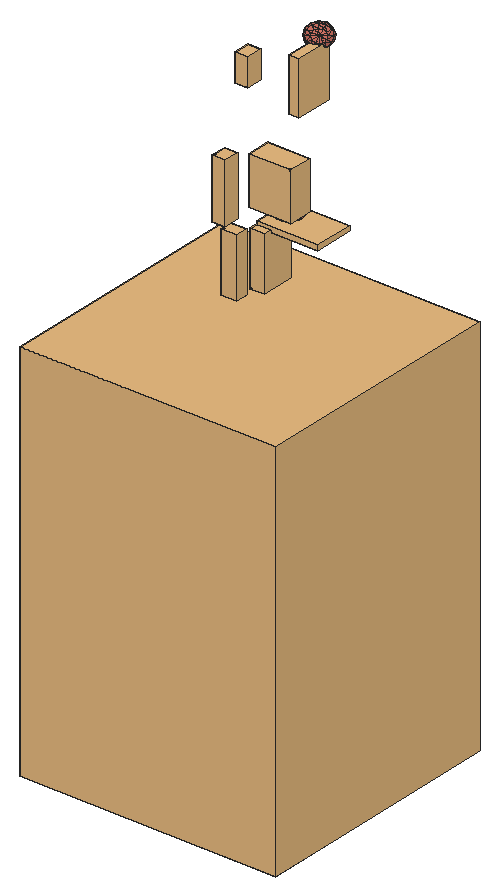
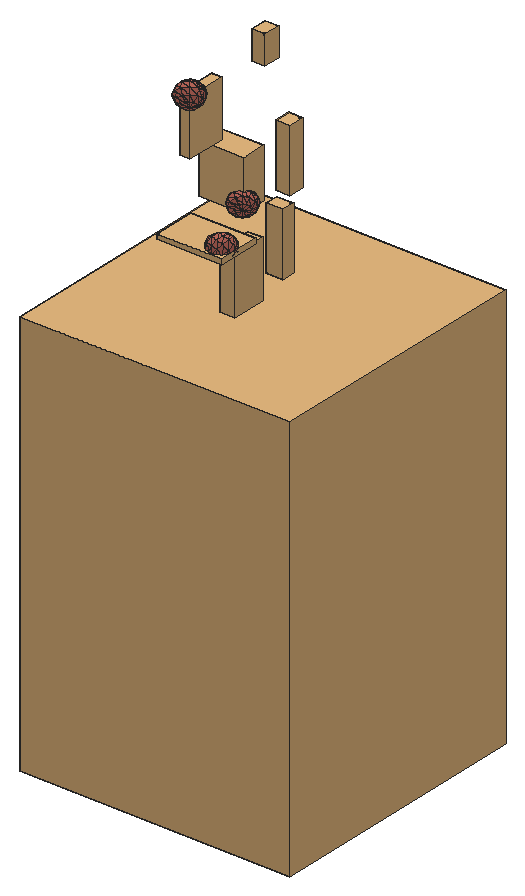
# SketchUp Ruby script. Lengths in inches.
U = 1.inch
M = Sketchup.active_model
def pt(a) = Geom::Point3d.new(a.map { |v| v * U })
def face(e, loops, mat)
  f = e.add_face(loops[0].map { |a| pt(a) })
  loops[1..].each { |l| e.add_face(l.map { |a| pt(a) }).erase! }
  f.material = f.back_material = mat if mat
  f
end
# faces: each face lists its corners as indices into pts; further lists are holes
def faces(e, pts, list, mat = nil) = list.each { |f| face(e, (f[0].is_a?(Array) ? f : [f]).map { |l| l.map { |i| pts[i] } }, mat) }
# xy, xz, yz: faces in a plane at the given z, y or x. An outline is a flat list of corners, or four numbers for a rectangle; further outlines are holes
def ring(l) = l.size == 4 ? [[l[0], l[1]], [l[2], l[1]], [l[2], l[3]], [l[0], l[3]]] : l.each_slice(2).to_a
def flat(e, list, mat, &to3) = list.each { |f| face(e, (f[0].is_a?(Array) ? f : [f]).map { |l| ring(l).map { |u, v| to3.(u, v) } }, mat) }
def xy(e, z, list, mat = nil) = flat(e, list, mat) { |x, y| [x, y, z] }
def xz(e, y, list, mat = nil) = flat(e, list, mat) { |x, z| [x, y, z] }
def yz(e, x, list, mat = nil) = flat(e, list, mat) { |y, z| [x, y, z] }
def lines(e, pts, list) = list.each { |a, b| e.add_line(pt(pts[a]), pt(pts[b])) }
# prism: a flat outline (further loops are holes) pulled along v
def prism(e, loops, v, mat = nil)
  f = face(e, loops, mat); d = Geom::Vector3d.new(v.map { |x| x * U })
  f.pushpull(f.normal.samedirection?(d) ? d.length : -d.length)
end
def box(e, o, s, mat = nil) = prism(e, [[o, [o[0] + s[0], o[1], o[2]], [o[0] + s[0], o[1] + s[1], o[2]], [o[0], o[1] + s[1], o[2]]]], [0, 0, s[2]], mat)
def at(x, y, z, deg = 0) = Geom::Transformation.translation(pt([x, y, z])) * Geom::Transformation.rotation(ORIGIN, Z_AXIS, deg.degrees)
def axes(o, x, y, z) = Geom::Transformation.new([*x, 0, *y, 0, *z, 0, *pt(o).to_a, 1])
def part(name) = M.definitions.add(name)
# library, detail: a bought-in or finely detailed component or shape, given as its bounding box
def library(name, o, s) = part(name).tap { |d| box(d.entities, o, s) }
def detail(e, o, s) = box(e.add_group.entities, o, s)
def put(e, d, t, mat = nil) = e.add_instance(d, t).tap { |i| i.material = mat if mat }
def group(e, t, mat = nil) = e.add_group.tap { |g| g.transformation = t; g.material = mat if mat }.entities
root = M.entities
M.materials.add("green").color = [174, 139, 102]
M.materials.add("st tile").color = [196, 179, 155]
M.materials.add("vio").color = [206, 114, 100]
c1 = library("3DGeom~165_Defintion",[-129.92,-500,-108.02],[259.84,1000,216.04])
c2 = part("3DGeom~166_Defintion")
p = [[102.48,500,-82.55],[119.68,491.3,-106.9],[111.55,493.01,-108.02],[102.48,500,-82.55],[111.55,493.01,-108.02],[104.2,495.34,-104.9],
  [102.48,500,-82.55],[126.4,490.68,-101.84],[119.68,491.3,-106.9],[102.48,500,-82.55],[104.2,495.34,-104.9],[99.59,497.67,-98.37],
  [102.48,500,-82.55],[129.92,491.3,-94.2],[126.4,490.68,-101.84],[102.48,500,-82.55],[99.59,497.67,-98.37],[98.96,499.375,-90.19],
  [102.48,500,-82.55],[129.29,493.01,-86.02],[129.92,491.3,-94.2],[102.48,500,-82.55],[124.6875,495.34,-79.5],[129.29,493.01,-86.02],
  [102.48,500,-82.55],[117.33,497.67,-76.375],[124.6875,495.34,-79.5],[102.48,500,-82.55],[109.21,499.375,-77.49],[117.33,497.67,-76.375],
  [-108.37,-495.57,69.37],[-118.11,-500,95.38],[-120.78,-498.52,79.375],[-93.3,-494.09,75.36],[-118.11,-500,95.38],[-108.37,-495.57,69.37],
  [-108.37,-495.57,69.37],[-120.78,-498.52,79.375],[-115.95,-497.04,72.67],[-93.3,-494.09,75.36],[-108.37,-495.57,69.37],[-100.08,-494.49,70.35],
  [-90.63,-495.57,91.37],[-118.11,-500,95.38],[-93.3,-494.09,75.36],[-90.63,-495.57,91.37],[-93.3,-494.09,75.36],[-89.84,-494.49,83.05],
  [-118.11,-500,95.38],[-121.57,-499.6,87.6875],[-120.78,-498.52,79.375],[-103.04,-498.52,101.375],[-118.11,-500,95.38],[-90.63,-495.57,91.37],
  [-103.04,-498.52,101.375],[-90.63,-495.57,91.37],[-95.46,-497.04,98.07],[-118.11,-500,95.38],[-103.04,-498.52,101.375],[-111.33,-499.6,100.39]]
faces(c2.entities,p,[[0,1,2],[3,4,5],[6,7,8],[9,10,11],[12,13,14],[15,16,17],[18,19,20],[21,22,23],
  [24,25,26],[27,28,29],[30,31,32],[33,34,35],[36,37,38],[39,40,41],[42,43,44],[45,46,47],
  [48,49,50],[51,52,53],[54,55,56],[57,58,59]],"green")
c3 = library("3DGeom~177_Defintion",[-102.18,-500,-134.58],[204.36,1000,269.16])
c4 = part("3DGeom~178_Defintion")
p = [[77.2,500,-106.58],[95.25,490.68,-131.46],[87.43,491.3,-134.58],[77.2,500,-106.58],[87.43,491.3,-134.58],[79.3,493.01,-133.53],
  [77.2,500,-106.58],[79.3,493.01,-133.53],[73.02,495.34,-128.6],[77.2,500,-106.58],[100.64,491.3,-125],[95.25,490.68,-131.46],
  [77.2,500,-106.58],[73.02,495.34,-128.6],[70.28,497.67,-121.1],[77.2,500,-106.58],[102.18,493.01,-116.9375],[100.64,491.3,-125],
  [77.2,500,-106.58],[70.28,497.67,-121.1],[71.81,499.375,-113.04],[77.2,500,-106.58],[99.43,495.34,-109.4375],[102.18,493.01,-116.9375],
  [77.2,500,-106.58],[93.15,497.67,-104.5],[99.43,495.34,-109.4375],[77.2,500,-106.58],[85.02,499.375,-103.46],[93.15,497.67,-104.5],
  [-70.48,-494.09,97.03],[-86.6,-495.57,95.18],[-78.34,-494.49,93.96],[-86.6,-495.57,95.18],[-89.2,-500,122.83],[-95.96,-498.52,108.09],
  [-70.48,-494.09,97.03],[-89.2,-500,122.83],[-86.6,-495.57,95.18],[-86.6,-495.57,95.18],[-95.96,-498.52,108.09],[-93.05,-497.04,100.35],
  [-63.72,-495.57,111.78],[-89.2,-500,122.83],[-70.48,-494.09,97.03],[-63.72,-495.57,111.78],[-70.48,-494.09,97.03],[-65.13,-494.49,103.55],
  [-89.2,-500,122.83],[-94.55,-499.6,116.32],[-95.96,-498.52,108.09],[-73.08,-498.52,124.68],[-89.2,-500,122.83],[-63.72,-495.57,111.78],
  [-73.08,-498.52,124.68],[-63.72,-495.57,111.78],[-66.63,-497.04,119.51],[-89.2,-500,122.83],[-73.08,-498.52,124.68],[-81.34,-499.6,125.9]]
faces(c4.entities,p,[[0,1,2],[3,4,5],[6,7,8],[9,10,11],[12,13,14],[15,16,17],[18,19,20],[21,22,23],
  [24,25,26],[27,28,29],[30,31,32],[33,34,35],[36,37,38],[39,40,41],[42,43,44],[45,46,47],
  [48,49,50],[51,52,53],[54,55,56],[57,58,59]],"green")
c5 = library("3DGeom~138_Defintion",[-301.73,-500,-131.06],[603.46,1000,262.12])
c6 = part("3DGeom~139_Defintion")
p = [[272.8,-500,-99.27],[285.64,-496.58,-110.875],[273.61,-494.75,-82.625],[285.64,-496.58,-110.875],[272.8,-500,-99.27],[278.1,-499.36,-106.75],
  [273.61,-494.75,-82.625],[285.64,-496.58,-110.875],[287.25,-486.08,-77.6],[285.64,-496.58,-110.875],[293.39,-492.38,-110.55],[299.28,-487.9,-105.84],
  [300.09,-482.66,-89.21],[285.64,-496.58,-110.875],[299.28,-487.9,-105.84],[287.25,-486.08,-77.6],[285.64,-496.58,-110.875],[300.09,-482.66,-89.21],
  [300.09,-482.66,-89.21],[299.28,-487.9,-105.84],[301.73,-484.35,-98.03],[272.8,-500,-99.27],[273.61,-494.75,-82.625],[271.16,-498.3125,-90.4375],
  [287.25,-486.08,-77.6],[300.09,-482.66,-89.21],[294.79,-483.3,-81.72],[273.61,-494.75,-82.625],[287.25,-486.08,-77.6],[279.5,-490.28,-77.93],
  [-291.23,494.98,97.6],[-301.04,485.9375,118.13],[-296.26,485.84,125.99],[-291.23,494.98,97.6],[-296.26,485.84,125.99],[-288.67,487.64,130.72],
  [-291.23,494.98,97.6],[-301.73,487.91,109.26],[-301.04,485.9375,118.13],[-291.23,494.98,97.6],[-288.67,487.64,130.72],[-280.29,490.86,131.0625],
  [-291.23,494.98,97.6],[-298.14,491.22,101.74],[-301.73,487.91,109.26],[-291.23,494.98,97.6],[-280.29,490.86,131.0625],[-273.38,494.625,126.92],
  [-291.23,494.98,97.6],[-273.38,494.625,126.92],[-269.79,497.9375,119.41],[-291.23,494.98,97.6],[-270.48,499.9,110.54],[-275.26,500,102.68],
  [-291.23,494.98,97.6],[-275.26,500,102.68],[-282.85,498.2,97.95],[-291.23,494.98,97.6],[-269.79,497.9375,119.41],[-270.48,499.9,110.54]]
faces(c6.entities,p,[[0,1,2],[3,4,5],[6,7,8],[9,10,11],[12,13,14],[15,16,17],[18,19,20],[21,22,23],
  [24,25,26],[27,28,29],[30,31,32],[33,34,35],[36,37,38],[39,40,41],[42,43,44],[45,46,47],
  [48,49,50],[51,52,53],[54,55,56],[57,58,59]],"green")
c7 = part("3DGeom~203_Defintion")
p = [[282.28,-215.46,-337.03],[49.88,-186.59,-454.85],[87.7,0,-500],[282.28,-215.46,-337.03],[325.95,0,-389.16],[-174.05,0,-476.86],
  [-195.89,107.73,-450.79],[49.88,186.59,-454.85],[325.95,0,-389.16],[-195.89,-107.73,-450.79],[-389.16,0,-325.95],[-389.16,0,-325.95],
  [162.97,-373.1875,-194.58],[-53.44,-323.1875,-331.49],[162.97,-373.1875,-194.58],[282.28,-215.46,-337.03],[325.95,0,-389.16],[282.28,215.46,-337.03],
  [-255.54,186.59,-379.57],[-255.54,186.59,-379.57],[-53.44,323.19,-331.49],[282.28,215.46,-337.03],[-53.44,323.19,-331.49],[-255.54,-186.59,-379.57],
  [-389.16,0,-325.95],[-255.54,186.59,-379.57],[-389.16,0,-325.95],[439.04,-186.59,-128.9],[282.28,-215.46,-337.03],[325.95,0,-389.16],
  [476.86,0,-174.05],[282.28,215.46,-337.03],[-194.58,-373.1875,-162.97],[-337.03,-215.46,-282.28],[-255.54,-186.59,-379.57],[-255.54,-186.59,-379.57],
  [-53.44,-323.1875,-331.49],[-255.54,-186.59,-379.57],[-337.03,-215.46,-282.28],[-389.16,0,-325.95],[-337.03,215.46,-282.28],[-255.54,186.59,-379.57],
  [-53.44,323.19,-331.49],[-255.54,186.59,-379.57],[-337.03,215.46,-282.28],[335.72,-323.19,-5.54],[162.97,-373.1875,-194.58],[439.04,186.59,-128.9],
  [162.97,373.1875,-194.58],[282.28,215.46,-337.03],[-53.44,323.19,-331.49],[162.97,373.1875,-194.58],[0,-430.92,0],[-53.44,-323.1875,-331.49],
  [-53.44,-323.1875,-331.49],[162.97,-373.1875,-194.58],[-337.03,215.46,-282.28],[-194.58,373.1875,-162.97],[162.97,373.1875,-194.58],[-418.51,-186.59,-184.99],
  [-478.17,-107.73,-113.77],[-500,0,-87.7],[-478.17,107.73,-113.77],[-418.51,186.59,-184.99],[-335.72,-323.19,5.54],[-194.58,-373.1875,-162.97],
  [-335.72,-323.19,5.54],[-194.58,373.1875,-162.97],[194.58,-373.1875,162.97],[162.97,-373.1875,-194.58],[162.97,-373.1875,-194.58],[335.72,-323.19,-5.54],
  [162.97,373.1875,-194.58],[335.72,323.19,-5.54],[335.72,323.19,-5.54],[0,430.92,0],[-439.04,-186.59,128.9],[-335.72,-323.19,5.54],
  [-335.72,323.19,5.54],[-194.58,373.1875,-162.97],[478.17,-107.73,113.77],[500,0,87.7],[-162.97,-373.1875,194.58],[-335.72,-323.19,5.54],
  [-335.72,323.19,5.54],[418.51,-186.59,184.99],[478.17,107.73,113.77],[-476.86,0,174.05],[-439.04,186.59,128.9],[337.03,-215.46,282.28],
  [194.58,-373.1875,162.97],[418.51,186.59,184.99],[194.58,373.1875,162.97],[335.72,323.19,-5.54],[194.58,373.1875,162.97],[53.44,-323.19,331.49],
  [-335.72,323.19,5.54],[-162.97,373.1875,194.58],[-162.97,373.1875,194.58],[-282.28,-215.46,337.03],[-335.72,-323.19,5.54],[-162.97,-373.1875,194.58],
  [-282.28,-215.46,337.03],[-335.72,-323.19,5.54],[-162.97,373.1875,194.58],[389.16,0,325.95],[-325.95,0,389.16],[-282.28,-215.46,337.03],
  [-325.95,0,389.16],[-282.28,215.46,337.03],[-162.97,373.1875,194.58],[-282.28,215.46,337.03],[255.54,-186.59,379.57],[255.54,-186.59,379.57],
  [337.03,-215.46,282.28],[194.58,373.1875,162.97],[337.03,215.46,282.28],[337.03,215.46,282.28],[53.44,323.19,331.49],[-162.97,373.1875,194.58],
  [53.44,323.19,331.49],[-282.28,215.46,337.03],[-325.95,0,389.16],[-49.88,-186.59,454.85],[-282.28,-215.46,337.03],[-162.97,-373.1875,194.58],
  [-162.97,-373.1875,194.58],[53.44,-323.19,331.49],[53.44,323.19,331.49],[-162.97,373.1875,194.58],[-282.28,215.46,337.03],[255.54,-186.59,379.57],
  [255.54,186.59,379.57],[337.03,215.46,282.28],[53.44,323.19,331.49],[255.54,186.59,379.57],[195.89,-107.73,450.79],[255.54,-186.59,379.57],
  [389.16,0,325.95],[174.05,0,476.86],[389.16,0,325.95],[195.89,107.73,450.79],[389.16,0,325.95],[255.54,186.59,379.57],
  [389.16,0,325.95],[53.44,-323.19,331.49],[53.44,-323.19,331.49],[255.54,-186.59,379.57],[-49.88,186.59,454.85],[-87.7,0,500],
  [-325.95,0,389.16]]
faces(c7.entities,p,[[0,1,2],[3,2,4],[1,5,2],[2,5,6],[2,6,7],[8,2,7],[1,9,5],[5,9,10],
  [6,5,11],[12,13,1],[14,1,15],[13,9,1],[16,7,17],[7,6,18],[7,19,20],[21,7,22],
  [13,23,9],[9,23,24],[25,6,26],[27,28,29],[27,29,30],[30,29,31],[32,33,34],[32,35,36],
  [37,38,39],[40,41,39],[42,43,44],[45,46,28],[45,28,27],[30,31,47],[47,31,48],[49,50,51],
  [52,32,53],[52,54,55],[42,56,57],[58,42,57],[38,59,39],[59,60,39],[60,61,39],[61,62,39],
  [62,63,39],[63,40,39],[64,38,65],[66,59,38],[67,40,63],[68,52,69],[68,70,71],[47,72,73],
  [74,58,75],[58,57,75],[76,59,77],[76,60,59],[78,63,62],[79,63,78],[80,27,30],[80,30,81],
  [81,30,47],[82,32,52],[82,83,32],[75,57,84],[85,45,27],[85,27,80],[81,47,86],[86,47,73],
  [87,60,76],[87,61,60],[88,62,61],[78,62,88],[88,61,87],[89,90,45],[89,45,85],[86,73,91],
  [91,73,92],[93,75,94],[95,82,52],[95,52,68],[75,96,97],[94,75,98],[99,100,101],[102,76,103],
  [104,78,88],[80,81,105],[81,86,105],[85,80,105],[86,91,105],[106,76,107],[108,87,76],[109,88,87],
  [110,88,111],[112,95,68],[113,68,114],[91,115,116],[117,94,118],[94,119,120],[121,87,122],[89,85,105],
  [91,116,105],[123,124,125],[123,126,127],[128,129,130],[131,89,105],[116,132,105],[133,134,135],[136,137,138],
  [139,136,140],[141,139,142],[143,141,144],[136,123,145],[136,146,147],[128,130,148],[143,128,148],[149,150,124],
  [149,124,123],[148,130,150],[143,148,141],[148,150,149],[139,123,136],[141,148,149],[141,149,139],[139,149,123]],"vio")
c8 = library("3DGeom~86_Defintion",[-294.02,-500,-230.29],[588.04,1000,460.58])
c9 = part("3DGeom~87_Defintion")
p = [[-277.25,494.74,-178.13],[-259.65,461.52,-230.29],[-276.72,461.46,-224.28],[-277.25,494.74,-178.13],[-242.66,466.72,-229.15],[-277.25,494.74,-178.13],
  [-230.3,475.68,-221.18],[-277.25,494.74,-178.13],[-276.72,461.46,-224.28],[-289.3,466.57,-212.75],[-277.25,494.74,-178.13],[-225.89,485.99,-208.51],
  [-230.3,475.68,-221.18],[-277.25,494.74,-178.13],[-289.3,466.57,-212.75],[-294.02,475.47,-198.77],[-277.25,494.74,-178.13],[-230.61,494.89,-194.54],
  [-225.89,485.99,-208.51],[-277.25,494.74,-178.13],[-294.02,475.47,-198.77],[-289.61,485.79,-186.1],[-277.25,494.74,-178.13],[-243.1875,500,-183],
  [-230.61,494.89,-194.54],[-277.25,494.74,-178.13],[-260.26,499.95,-177],[-243.1875,500,-183],[274.19,-487.18,163.98],[243.1875,-498.77,172.64],
  [258.02,-494.08,163.86],[274.19,-487.18,163.98],[251.86,-484.5,230.17],[243.1875,-498.77,172.64],[294.02,-474.24,188.41],[251.86,-484.5,230.17],
  [274.19,-487.18,163.98],[294.02,-474.24,188.41],[274.19,-487.18,163.98],[287.36,-479.92,172.97],[243.1875,-498.77,172.64],[232.02,-497.43,205.74],
  [233.67,-500,187.97],[243.1875,-498.77,172.64],[251.86,-484.5,230.17],[232.02,-497.43,205.74],[282.85,-472.9,221.51],[251.86,-484.5,230.17],
  [294.02,-474.24,188.41],[282.85,-472.9,221.51],[294.02,-474.24,188.41],[292.37,-471.67,206.18],[251.86,-484.5,230.17],[238.68,-491.76,221.18],
  [232.02,-497.43,205.74],[251.86,-484.5,230.17],[282.85,-472.9,221.51],[268.02,-477.6,230.29]]
faces(c9.entities,p,[[0,1,2],[3,4,1],[5,6,4],[7,8,9],[10,11,12],[13,14,15],[16,17,18],[19,20,21],
  [22,23,24],[25,26,27],[28,29,30],[31,32,33],[34,35,36],[37,38,39],[40,41,42],[43,44,45],
  [46,47,48],[49,50,51],[52,53,54],[55,56,57]],"green")
c10 = part("3DGeom~231_Defintion")
p = [[55.77,-247.26,-406.4],[-282.99,-160.1875,-370.7],[-76.91,-70.8125,-490.14],[264.6875,-115.27,-405.72],[-380.05,9.05,-329.48],[149.78,37.54,-478.25],
  [-188.98,124.61,-442.55],[402.68,47.61,-296.34],[52.72,206.77,-437.03],[336.34,135.83,-338.21],[402.68,47.61,-296.34],[336.34,135.83,-338.21],
  [-433.25,149.375,-185.58],[-433.25,149.375,-185.58],[-250.42,286.64,-276.38],[-250.42,286.64,-276.38],[336.34,135.83,-338.21],[280.3,233.54,-314.41],
  [-250.42,286.64,-276.38],[-0.48,347.1,-293.125],[280.3,233.54,-314.41],[-0.48,347.1,-293.125],[173.51,-357.45,-213.76],[-168.09,-312.99,-298.18],
  [55.77,-247.26,-406.4],[366.65,-210.7,-238.9],[173.51,-357.45,-213.76],[-168.09,-312.99,-298.18],[366.65,-210.7,-238.9],[461.55,-7.49,-200.02],
  [366.65,-210.7,-238.9],[264.6875,-115.27,-405.72],[264.6875,-115.27,-405.72],[402.68,47.61,-296.34],[-168.09,-312.99,-298.18],[-413.24,-206.64,-151.93],
  [-282.99,-160.1875,-370.7],[-282.99,-160.1875,-370.7],[-469.28,-108.93,-128.14],[-282.99,-160.1875,-370.7],[-380.05,9.05,-329.48],[336.34,135.83,-338.21],
  [432.77,197.72,-107.55],[280.3,233.54,-314.41],[-380.05,9.05,-329.48],[-500,-27.91,-45.05],[-380.05,9.05,-329.48],[-433.25,149.375,-185.58],
  [249.58,314.55,-231.33],[280.3,233.54,-314.41],[-0.48,347.1,-293.125],[249.58,314.55,-231.33],[-66.125,-408.42,-131.35],[-346.9,-294.86,-110.06],
  [-168.09,-312.99,-298.18],[173.51,-357.45,-213.76],[-168.09,-312.99,-298.18],[-168.09,-312.99,-298.18],[-346.9,-294.86,-110.06],[-0.48,347.1,-293.125],
  [-250.42,286.64,-276.38],[-244.75,371.86,-36.15],[249.58,314.55,-231.33],[4.42,420.91,-85.08],[-250.42,286.64,-276.38],[-428.35,223.18,22.47],
  [-250.42,286.64,-276.38],[-244.75,371.86,-36.15],[428.35,-223.18,-22.47],[173.51,-357.45,-213.76],[497.17,-14.7,-75.0625],[252.41,357.17,-111.21],
  [249.58,314.55,-231.33],[252.41,357.17,-111.21],[244.75,-371.86,36.15],[173.51,-357.45,-213.76],[244.75,-371.86,36.15],[173.51,-357.45,-213.76],
  [-497.17,14.7,75.0625],[-432.77,-197.72,107.55],[-4.42,-420.91,85.08],[-288.04,-349.96,-13.74],[244.75,-371.86,36.15],[-346.9,-294.86,-110.06],
  [288.04,349.96,13.74],[252.41,357.17,-111.21],[66.12,408.42,131.35],[288.04,349.96,13.74],[252.41,357.17,-111.21],[-288.04,-349.96,-13.74],
  [500,27.91,45.05],[469.28,108.93,128.14],[413.24,206.64,151.93],[346.9,294.86,110.06],[-173.51,357.45,213.76],[-244.75,371.86,-36.15],
  [-366.65,210.7,238.9],[-244.75,371.86,-36.15],[-366.65,210.7,238.9],[-173.51,357.45,213.76],[433.25,-149.375,185.58],[-252.41,-357.17,111.22],
  [-288.04,-349.96,-13.74],[-252.41,-357.17,111.22],[288.04,349.96,13.74],[168.09,312.99,298.18],[346.9,294.86,110.06],[288.04,349.96,13.74],
  [168.09,312.99,298.18],[-461.55,7.49,200.02],[-366.65,210.7,238.9],[250.42,-286.64,276.38],[244.75,-371.86,36.15],[250.42,-286.64,276.38],
  [0.48,-347.1,293.125],[250.42,-286.64,276.38],[-252.41,-357.17,111.22],[-249.58,-314.55,231.33],[-249.58,-314.55,231.33],[-280.3,-233.54,314.41],
  [-280.3,-233.54,314.41],[-336.34,-135.83,338.21],[-402.68,-47.6,296.34],[-336.34,-135.83,338.21],[-402.68,-47.6,296.34],[168.09,312.99,298.18],
  [282.99,160.1875,370.7],[-249.58,-314.55,231.33],[380.05,-9.05,329.48],[-55.77,247.26,406.4],[-55.77,247.26,406.4],[168.09,312.99,298.18],
  [380.05,-9.05,329.48],[250.42,-286.64,276.38],[433.25,-149.375,185.58],[-366.65,210.7,238.9],[-402.68,-47.6,296.34],[-173.51,357.45,213.76],
  [-366.65,210.7,238.9],[-264.6875,115.27,405.72],[-173.51,357.45,213.76],[-55.77,247.26,406.4],[-52.72,-206.77,437.03],[-249.58,-314.55,231.33],
  [0.48,-347.1,293.125],[-280.3,-233.54,314.41],[-249.58,-314.55,231.33],[-366.65,210.7,238.9],[-402.68,-47.6,296.34],[-264.6875,115.27,405.72],
  [188.98,-124.61,442.55],[0.48,-347.1,293.125],[250.42,-286.64,276.38],[380.05,-9.05,329.48],[250.42,-286.64,276.38],[0.48,-347.1,293.125],
  [-402.68,-47.6,296.34],[-336.34,-135.83,338.21],[168.09,312.99,298.18],[76.91,70.8125,490.14],[168.09,312.99,298.18],[282.99,160.1875,370.7],
  [-149.78,-37.54,478.25],[282.99,160.1875,370.7],[380.05,-9.05,329.48],[282.99,160.1875,370.7]]
faces(c10.entities,p,[[0,1,2],[3,0,2],[2,1,4],[3,2,5],[2,4,6],[5,2,6],[7,3,5],[5,6,8],
  [9,5,8],[10,5,11],[6,4,12],[6,13,14],[8,6,15],[16,8,17],[8,18,19],[20,8,21],
  [22,23,24],[25,26,0],[0,27,1],[28,0,3],[29,30,31],[29,32,33],[34,35,36],[37,35,38],
  [39,38,40],[33,41,42],[41,43,42],[44,38,45],[46,45,47],[43,48,42],[49,50,51],[52,53,54],
  [55,52,56],[57,58,35],[29,33,42],[59,60,61],[62,59,63],[59,61,63],[64,47,65],[66,65,67],
  [68,69,30],[70,68,30],[70,30,29],[48,71,42],[72,63,73],[74,52,75],[68,76,77],[70,29,42],
  [47,45,78],[47,78,65],[35,58,79],[38,35,79],[80,81,52],[82,80,52],[52,81,83],[45,38,79],
  [71,84,42],[85,86,87],[88,63,86],[58,89,79],[90,70,42],[91,90,42],[92,91,42],[84,93,42],
  [93,92,42],[63,61,94],[63,94,86],[90,68,70],[78,45,79],[95,65,96],[97,98,99],[100,76,68],
  [90,100,68],[80,101,81],[102,103,79],[104,105,106],[107,86,108],[65,78,109],[65,109,110],[111,80,112],
  [100,113,76],[91,100,90],[109,78,79],[114,101,80],[115,114,80],[116,117,79],[118,119,79],[120,121,79],
  [122,109,79],[123,124,79],[93,125,126],[93,126,92],[114,127,101],[91,128,100],[92,128,91],[86,94,129],
  [86,130,131],[92,126,128],[132,133,134],[135,109,136],[137,138,139],[140,139,141],[142,143,144],[142,145,146],
  [147,148,149],[150,151,152],[153,150,154],[150,142,155],[139,156,157],[158,141,159],[160,159,161],[162,157,145],
  [162,145,142],[163,150,164],[139,157,162],[165,159,150],[141,139,162],[141,162,159],[159,162,142],[159,142,150]],"vio")
c11 = part("3DGeom~201_Defintion")
p = [[110.02,-100.74,-478.98],[-201.3,-79.76,-454.16],[-6.43,63.34,-500],[324.63,0,-387.59],[-294.01,-10.41,-411.12],[-167.01,183.46,-425.45],
  [324.63,0,-387.59],[190.15,189.47,-411.86],[190.15,189.47,-411.86],[151.15,-264.83,-368.01],[-134.06,-174.49,-442.02],[372.12,-189.47,-259.46],
  [372.12,-189.47,-259.46],[324.63,0,-387.59],[-342.22,-201.49,-286.63],[-342.22,-201.49,-286.63],[-110.3125,-269.23,-377.96],[-342.22,-201.49,-286.63],
  [-387.35,14.98,-324.43],[-387.35,14.98,-324.43],[-328.69,227.43,-275.3],[4.73,328.17,-325.78],[-328.69,227.43,-275.3],[190.15,189.47,-411.86],
  [4.73,328.17,-325.78],[452.25,100.74,-192.35],[324.63,0,-387.59],[190.15,189.47,-411.86],[190.15,189.47,-411.86],[335.79,264.83,-213.37],
  [335.79,264.83,-213.37],[190.15,189.47,-411.86],[4.73,328.17,-325.78],[-387.35,14.98,-324.43],[-294.01,-10.41,-411.12],[-342.22,-201.49,-286.63],
  [493.375,-63.34,-81.39],[372.12,-189.47,-259.46],[105.93,-384.95,-196.84],[-136.42,-338.58,-279.13],[-110.3125,-269.23,-377.96],[-110.3125,-269.23,-377.96],
  [151.15,-264.83,-368.01],[-136.42,-338.58,-279.13],[-342.22,-201.49,-286.63],[319.9,-328.17,-61.81],[151.15,-264.83,-368.01],[319.9,-328.17,-61.81],
  [151.15,-264.83,-368.01],[372.12,-189.47,-259.46],[4.73,328.17,-325.78],[-328.69,227.43,-275.3],[-181.96,378.94,-152.4],[175.21,384.95,-138.82],
  [-181.96,378.94,-152.4],[-456.32,-10.41,-217.32],[-328.69,227.43,-275.3],[-205.39,-363.96,-172.03],[-342.22,-201.49,-286.63],[-205.39,-363.96,-172.03],
  [-298.74,-338.58,-85.34],[-298.74,-338.58,-85.34],[-391.45,-269.23,-42.3],[-391.45,-269.23,-42.3],[-458.6875,-174.49,-54.43],[-482.43,-79.76,-118.5],
  [-13.53,-428.92,-11.33],[-448.15,183.46,-89.79],[-181.96,378.94,-152.4],[448.15,-183.46,89.79],[319.9,-328.17,-61.81],[458.6875,174.49,54.43],
  [335.79,264.83,-213.37],[335.79,264.83,-213.37],[391.45,269.23,42.3],[391.45,269.23,42.3],[181.96,-378.94,152.4],[181.96,-378.94,152.4],
  [319.9,-328.17,-61.81],[482.43,79.76,118.5],[-175.21,-384.95,138.82],[-298.74,-338.58,-85.34],[-181.96,378.94,-152.4],[-319.9,328.17,61.81],
  [13.53,428.92,11.33],[-319.9,328.17,61.81],[391.45,269.23,42.3],[298.74,338.58,85.34],[298.74,338.58,85.34],[-493.375,63.34,81.38],
  [-319.9,328.17,61.81],[-335.79,-264.83,213.37],[-391.45,-269.23,-42.3],[456.32,10.41,217.32],[328.69,-227.43,275.3],[181.96,-378.94,152.4],
  [328.69,-227.43,275.3],[-452.25,-100.74,192.35],[-391.45,-269.23,-42.3],[-391.45,-269.23,-42.3],[-335.79,-264.83,213.37],[-4.73,-328.17,325.78],
  [-4.73,-328.17,325.78],[181.96,-378.94,152.4],[-105.93,384.95,196.84],[298.74,338.58,85.34],[205.39,363.96,172.03],[342.22,201.49,286.63],
  [298.74,338.58,85.34],[-319.9,328.17,61.81],[-372.12,189.47,259.46],[-372.12,189.47,259.46],[-372.12,189.47,259.46],[205.39,363.96,172.03],
  [387.35,-14.98,324.43],[328.69,-227.43,275.3],[-190.15,-189.47,411.86],[-190.15,-189.47,411.86],[-4.73,-328.17,325.78],[167.01,-183.46,425.45],
  [-4.73,-328.17,325.78],[181.96,-378.94,152.4],[328.69,-227.43,275.3],[136.42,338.58,279.13],[342.22,201.49,286.63],[136.42,338.58,279.13],
  [-324.63,0,387.59],[-335.79,-264.83,213.37],[-372.12,189.47,259.46],[-324.63,0,387.59],[-372.12,189.47,259.46],[-151.15,264.83,368.01],
  [136.42,338.58,279.13],[-151.15,264.83,368.01],[-324.63,0,387.59],[-335.79,-264.83,213.37],[-190.15,-189.47,411.86],[-151.15,264.83,368.01],
  [-372.12,189.47,259.46],[-324.63,0,387.59],[294.01,10.41,411.12],[294.01,10.41,411.12],[387.35,-14.98,324.43],[136.42,338.58,279.13],
  [110.3125,269.23,377.96],[342.22,201.49,286.63],[136.42,338.58,279.13],[-151.15,264.83,368.01],[110.3125,269.23,377.96],[294.01,10.41,411.12],
  [201.3,79.76,454.16],[294.01,10.41,411.12],[342.22,201.49,286.63],[134.06,174.49,442.02],[342.22,201.49,286.63],[342.22,201.49,286.63],
  [6.43,-63.34,500],[-190.15,-189.47,411.86],[-110.03,100.74,478.98],[294.01,10.41,411.12]]
faces(c11.entities,p,[[0,1,2],[3,0,2],[2,1,4],[2,4,5],[6,2,7],[8,2,5],[9,10,0],[11,9,0],
  [12,0,13],[0,10,1],[4,1,14],[1,10,15],[10,16,17],[9,16,10],[5,4,18],[5,19,20],
  [21,5,22],[23,5,24],[25,26,27],[25,28,29],[30,31,32],[33,34,35],[36,37,26],[36,26,25],
  [38,39,40],[38,41,42],[16,43,44],[45,38,46],[47,48,49],[50,51,52],[30,32,53],[53,32,54],
  [55,33,35],[56,33,55],[39,57,58],[59,60,35],[61,62,35],[63,64,35],[64,65,35],[65,55,35],
  [66,57,39],[66,39,38],[56,55,67],[68,56,67],[69,70,37],[69,37,36],[67,55,65],[71,25,72],
  [71,73,74],[75,30,53],[76,66,38],[77,38,78],[79,36,25],[79,25,71],[80,57,66],[80,81,57],
  [82,67,83],[84,54,85],[53,54,84],[86,53,87],[88,53,84],[89,65,64],[67,65,89],[90,67,89],
  [91,81,80],[91,92,81],[93,69,36],[93,36,79],[94,95,70],[96,70,69],[97,64,98],[89,64,97],
  [97,99,100],[101,80,66],[102,66,103],[84,85,104],[105,84,106],[106,84,104],[71,74,107],[74,108,107],
  [79,71,107],[109,89,110],[104,85,111],[112,89,97],[108,113,107],[114,115,69],[114,69,93],[93,79,107],
  [116,91,80],[117,80,118],[119,120,121],[119,121,122],[106,123,124],[106,104,125],[126,97,127],[128,97,129],
  [104,130,131],[132,104,133],[134,135,136],[114,93,107],[137,138,139],[140,119,122],[141,122,142],[143,144,145],
  [146,147,148],[149,114,107],[150,151,152],[153,150,154],[144,153,155],[156,157,120],[156,120,119],[137,139,158],
  [144,137,158],[144,158,153],[158,139,157],[150,119,159],[158,157,156],[150,156,119],[153,158,156],[153,156,150]],"vio")
c12 = library("3DGeom~51_Defintion",[-354.35,-500,-93.25],[708.7,1000,186.5])
c13 = part("3DGeom~52_Defintion")
p = [[-330.32,495.99,-90.07],[-337.71,491.72,-93.25],[-345.49,487.36,-91.53],[-330.32,495.99,-90.07],[-345.49,487.36,-91.53],[-351.58,484.07,-85.375],
  [-330.32,495.99,-90.07],[-351.58,484.07,-85.375],[-354.35,482.74,-76.44],[-330.32,495.99,-90.07],[-354.35,482.74,-76.44],[-353.05,483.72,-67.125],
  [-330.32,495.99,-90.07],[-353.05,483.72,-67.125],[-348.04,486.75,-59.91],[-330.32,495.99,-90.07],[-348.04,486.75,-59.91],[-340.65,491.02,-56.74],
  [-330.32,495.99,-90.07],[-340.65,491.02,-56.74],[-332.87,495.38,-58.46],[-330.32,495.99,-90.07],[-332.87,495.38,-58.46],[-326.78,498.67,-64.61],
  [-330.32,495.99,-90.07],[-326.78,498.67,-64.61],[-324.02,500,-73.54],[-330.32,495.99,-90.07],[-324.02,500,-73.54],[-325.3125,499.02,-82.86],
  [349.875,-495.14,64.65],[332.69,-500,61.93],[341.95,-498.4,61.14],[332.69,-500,61.93],[349.875,-495.14,64.65],[319.79,-497.07,74.47],
  [332.69,-500,61.93],[319.79,-497.07,74.47],[324.58,-499.51,66.81],[319.79,-497.07,74.47],[349.875,-495.14,64.65],[324.08,-489.29,89.73],
  [324.08,-489.29,89.73],[349.875,-495.14,64.65],[341.27,-484.43,92.46],[341.27,-484.43,92.46],[349.875,-495.14,64.65],[354.16,-487.36,79.92],
  [349.875,-495.14,64.65],[354.35,-491.1,71.52],[354.16,-487.36,79.92],[319.79,-497.07,74.47],[324.08,-489.29,89.73],[319.61,-493.33,82.86],
  [341.27,-484.43,92.46],[354.16,-487.36,79.92],[349.38,-484.91,87.58],[324.08,-489.29,89.73],[341.27,-484.43,92.46],[332.01,-486.03,93.25]]
faces(c13.entities,p,[[0,1,2],[3,4,5],[6,7,8],[9,10,11],[12,13,14],[15,16,17],[18,19,20],[21,22,23],
  [24,25,26],[27,28,29],[30,31,32],[33,34,35],[36,37,38],[39,40,41],[42,43,44],[45,46,47],
  [48,49,50],[51,52,53],[54,55,56],[57,58,59]],"green")
c14 = library("3DGeom~187_Defintion",[-331.51,-500,-331.51],[663.02,1000,663.02])
c15 = library("3DGeom~49_Defintion",[-249.27,-500,-442.2],[498.54,1000,884.4])
c16 = part("3DGeom~50_Defintion")
p = [[-222.48,-492.22,-439.3125],[-238.52,-481.53,-439.75],[-230.08,-486.5,-442.2],[-238.52,-481.53,-439.75],[-222.48,-492.22,-439.3125],[-249.27,-478.62,-422.75],
  [-238.52,-481.53,-439.75],[-249.27,-478.62,-422.75],[-245.54,-478.65,-432.64],[-227.92,-497.09,-404.87],[-222.48,-492.22,-439.3125],[-217.17,-500,-421.87],
  [-222.48,-492.22,-439.3125],[-217.75,-497.16,-431.875],[-217.17,-500,-421.87],[-243.96,-486.4,-405.31],[-222.48,-492.22,-439.3125],[-227.92,-497.09,-404.87],
  [-249.27,-478.62,-422.75],[-222.48,-492.22,-439.3125],[-243.96,-486.4,-405.31],[-249.27,-478.62,-422.75],[-243.96,-486.4,-405.31],[-248.6875,-481.46,-412.75],
  [-227.92,-497.09,-404.87],[-217.17,-500,-421.87],[-220.89,-499.97,-411.99],[-243.96,-486.4,-405.31],[-227.92,-497.09,-404.87],[-236.36,-492.12,-402.43],
  [245.19,493.0625,414.62],[236.94,497.78,411.0625],[226.73,500,411.68],[245.19,493.0625,414.62],[226.73,500,411.68],[217.29,499.13,416.31],
  [245.19,493.0625,414.62],[222.29,479.16,442.2],[232.5,476.9375,441.58],[245.19,493.0625,414.62],[241.9375,477.81,436.95],[245.19,493.0625,414.62],
  [241.9375,477.81,436.95],[248.08,481.53,429.5625],[245.19,493.0625,414.62],[214.04,483.875,438.65],[245.19,493.0625,414.62],[248.08,481.53,429.5625],
  [249.27,487.12,421.39],[245.19,493.0625,414.62],[209.96,489.82,431.875],[245.19,493.0625,414.62],[211.15,495.41,423.7],[209.96,489.82,431.875],
  [245.19,493.0625,414.62],[217.29,499.13,416.31],[211.15,495.41,423.7]]
faces(c16.entities,p,[[0,1,2],[3,4,5],[6,7,8],[9,10,11],[12,13,14],[15,16,17],[18,19,20],[21,22,23],
  [24,25,26],[27,28,29],[30,31,32],[33,34,35],[36,37,38],[39,38,40],[41,42,43],[44,45,37],
  [46,47,48],[49,50,45],[51,52,53],[54,55,56]],"green")
c17 = library("3DGeom~63_Defintion",[-323.2,-41,-500],[646.4,82,1000])
c18 = part("3DGeom~64_Defintion")
p = [[311.67,-40.04,-491.9],[306.7,-29.34,-500],[319.92,-38.4,-478.58],[306.7,-29.34,-500],[311.67,-40.04,-491.9],[308.29,-35.77,-497.38],
  [319.92,-38.4,-478.58],[306.7,-29.34,-500],[323.2,-26.06,-473.36],[306.7,-29.34,-500],[307.3125,-22.47,-499.05],[309.97,-17,-494.78],
  [318.22,-15.36,-481.47],[306.7,-29.34,-500],[309.97,-17,-494.78],[323.2,-26.06,-473.36],[306.7,-29.34,-500],[318.22,-15.36,-481.47],
  [318.22,-15.36,-481.47],[309.97,-17,-494.78],[313.97,-14.4,-488.35],[311.67,-40.04,-491.9],[319.92,-38.4,-478.58],[315.93,-41,-485.02],
  [323.2,-26.06,-473.36],[318.22,-15.36,-481.47],[321.6,-19.63,-475.98],[319.92,-38.4,-478.58],[323.2,-26.06,-473.36],[322.58,-32.93,-474.31],
  [-323.2,26.33,486.21],[-308.11,14.4,494.77],[-301.1875,16.87,498],[-323.2,26.33,486.21],[-315.3,15.5,491.1],[-308.11,14.4,494.77],
  [-323.2,26.33,486.21],[-320.82,19.86,487.96],[-315.3,15.5,491.1],[-323.2,26.33,486.21],[-301.1875,16.87,498],[-296.38,22.24,499.91],
  [-323.2,26.33,486.21],[-296.38,22.24,499.91],[-294.98,29.07,500],[-323.2,26.33,486.21],[-310.07,41,491.4375],[-316.99,38.53,488.21],
  [-323.2,26.33,486.21],[-316.99,38.53,488.21],[-321.8,33.16,486.3],[-323.2,26.33,486.21],[-297.36,35.54,498.24],[-302.88,39.9,495.11],
  [-323.2,26.33,486.21],[-302.88,39.9,495.11],[-310.07,41,491.4375],[-323.2,26.33,486.21],[-294.98,29.07,500],[-297.36,35.54,498.24]]
faces(c18.entities,p,[[0,1,2],[3,4,5],[6,7,8],[9,10,11],[12,13,14],[15,16,17],[18,19,20],[21,22,23],
  [24,25,26],[27,28,29],[30,31,32],[33,34,35],[36,37,38],[39,40,41],[42,43,44],[45,46,47],
  [48,49,50],[51,52,53],[54,55,56],[57,58,59]],"green")
g1 = group(root,at(15.3125,38.42,26.21))
put(g1,c1,axes([-0.88,-0.16,7.92],[0,0.00091,0],[0,0,-0.00091],[-0.00091,0,0]),"green")
put(g1,c2,axes([-0.88,-0.16,7.92],[0,0.00091,0],[0,0,-0.00091],[-0.00091,0,0]),"green")
g2 = group(root,at(15.3125,38.42,26.21))
put(g2,c3,axes([-0.83,-0.05,6.86],[0,0.00091,0],[0,0,-0.00091],[-0.00091,0,0]),"green")
put(g2,c4,axes([-0.83,-0.05,6.86],[0,0.00091,0],[0,0,-0.00091],[-0.00091,0,0]),"green")
g3 = group(root,at(15.3125,38.42,26.21))
put(g3,c5,axes([-0.82,0.64,6.68],[0,0.00083,0],[0,0,-0.00083],[-0.00083,0,0]),"green")
put(g3,c6,axes([-0.82,0.64,6.68],[0,0.00083,0],[0,0,-0.00083],[-0.00083,0,0]),"green")
g4 = group(root,at(15.3125,38.42,26.21))
put(g4,c7,axes([-0.82,0.61,7.6],[0,0.00038,0],[0,0,-0.00038],[-0.00038,0,0]),"vio")
g5 = group(root,at(15.3125,38.42,26.21))
put(g5,c8,axes([-0.79,0.17,9.47],[0,0.00042,0],[0,0,-0.00042],[-0.00042,0,0]),"green")
put(g5,c9,axes([-0.79,0.17,9.47],[0,0.00042,0],[0,0,-0.00042],[-0.00042,0,0]),"green")
g6 = group(root,at(15.3125,38.42,26.21))
put(g6,c10,axes([-0.74,0.9,7.125],[0,0.00039,0],[0,0,-0.00039],[-0.00039,0,0]),"vio")
g7 = group(root,at(15.3125,38.42,26.21))
put(g7,c11,axes([-0.73,1.46,9.35],[0,0.00039,0],[0,0,-0.00039],[-0.00039,0,0]),"vio")
g8 = group(root,at(15.3125,38.42,26.21))
put(g8,c12,axes([-0.66,1.17,8.92],[0,0.00081,0],[0,0,-0.00081],[-0.00081,0,0]),"green")
put(g8,c13,axes([-0.66,1.17,8.92],[0,0.00081,0],[0,0,-0.00081],[-0.00081,0,0]),"green")
g9 = group(root,at(15.3125,38.42,26.21))
put(g9,c14,axes([-0.6,-0.03,2.99],[0,0.0059,0],[0,0,-0.0059],[-0.0059,0,0]),"st tile")
g10 = group(root,at(15.3125,38.42,26.21))
put(g10,c15,axes([-0.52,0.44,7.84],[0,0.00073,0],[0,0,-0.00073],[-0.00073,0,0]),"green")
put(g10,c16,axes([-0.52,0.44,7.84],[0,0.00073,0],[0,0,-0.00073],[-0.00073,0,0]),"green")
g11 = group(root,at(15.3125,38.42,26.21))
put(g11,c17,axes([-0.46,0.82,7.1],[0,0.00094,0],[0,0,-0.00094],[-0.00094,0,0]),"green")
put(g11,c18,axes([-0.46,0.82,7.1],[0,0.00094,0],[0,0,-0.00094],[-0.00094,0,0]),"green")
